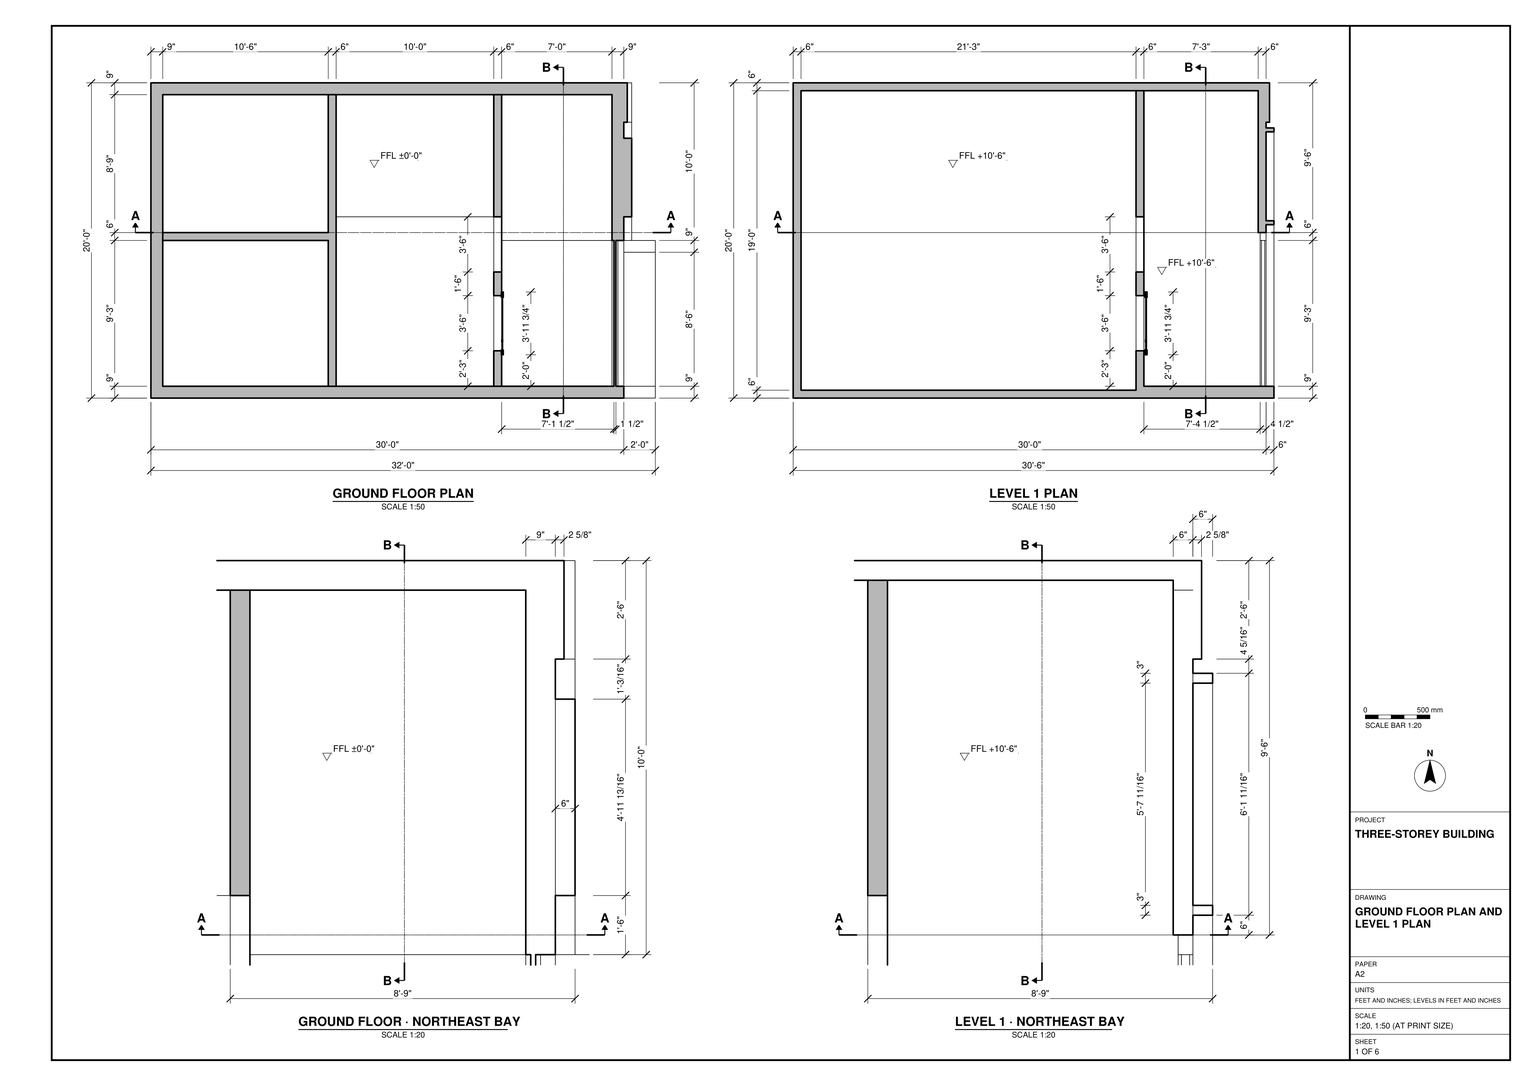
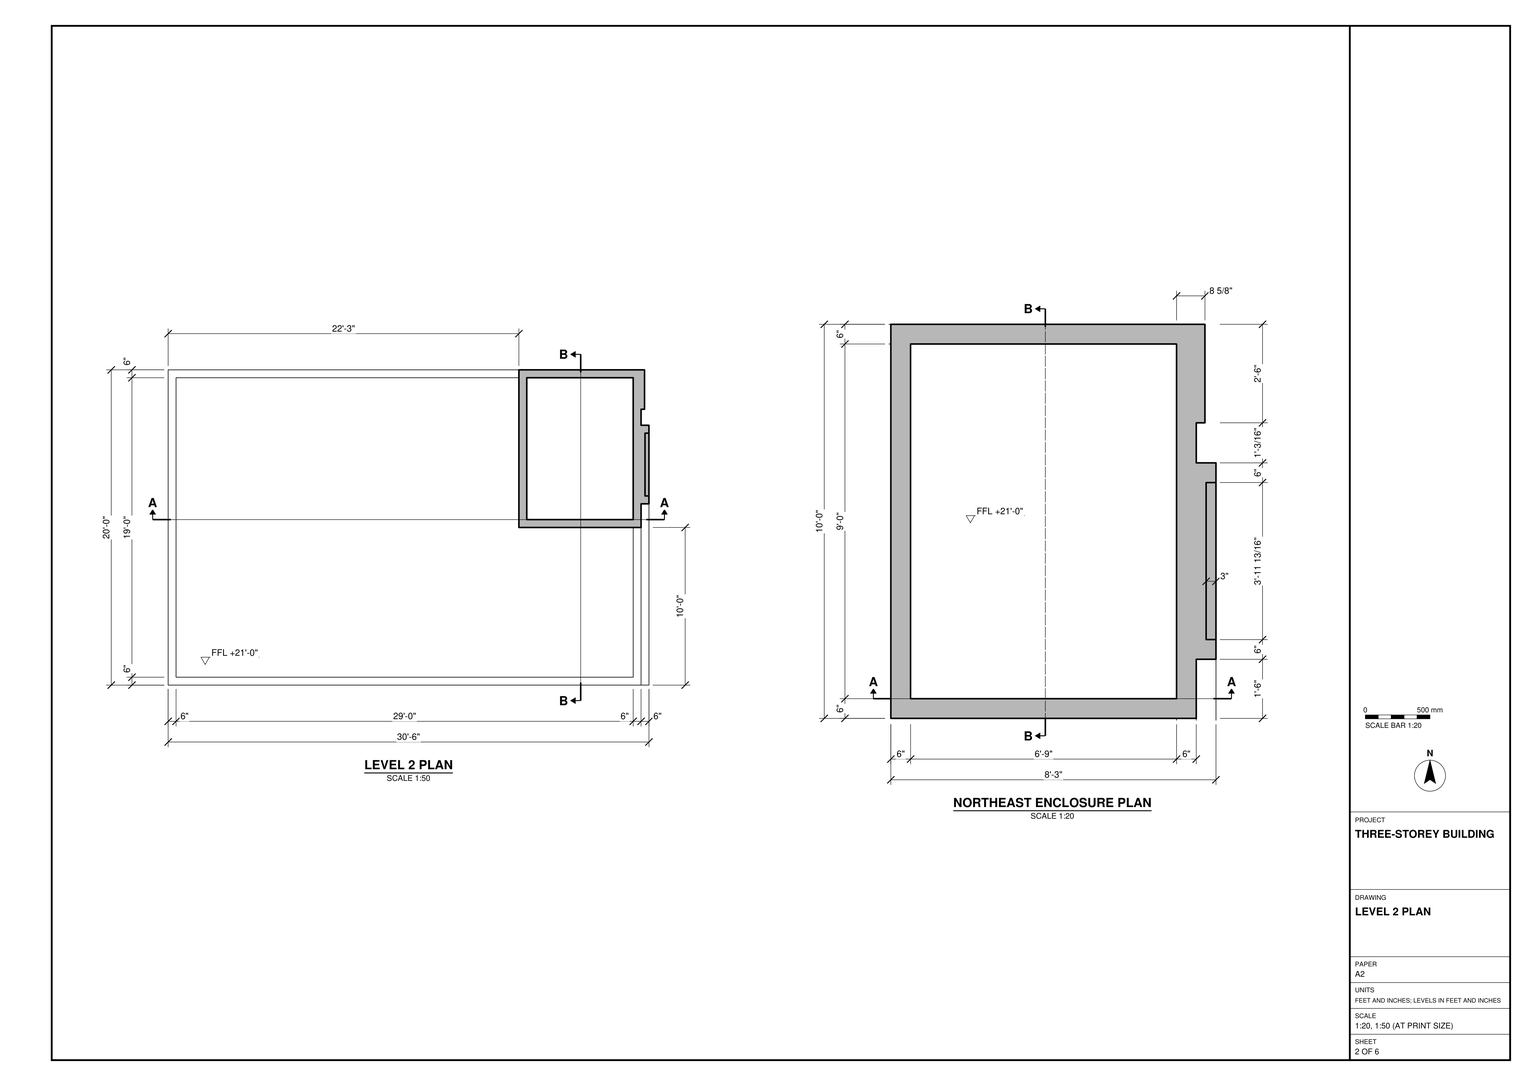
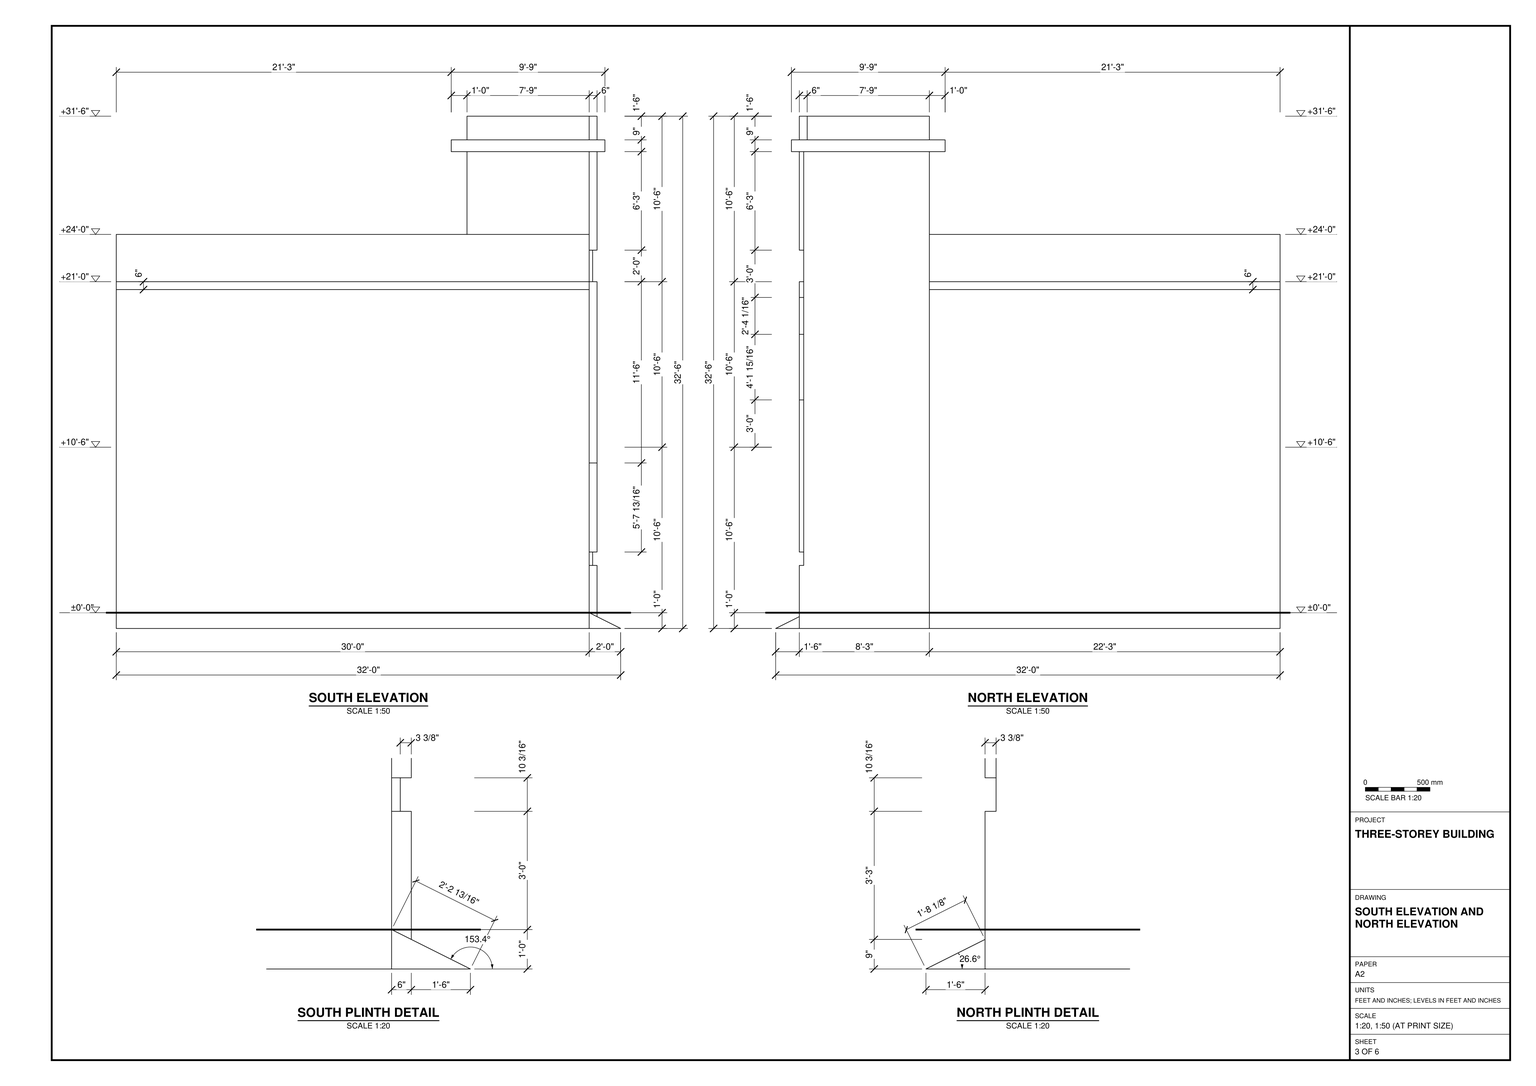
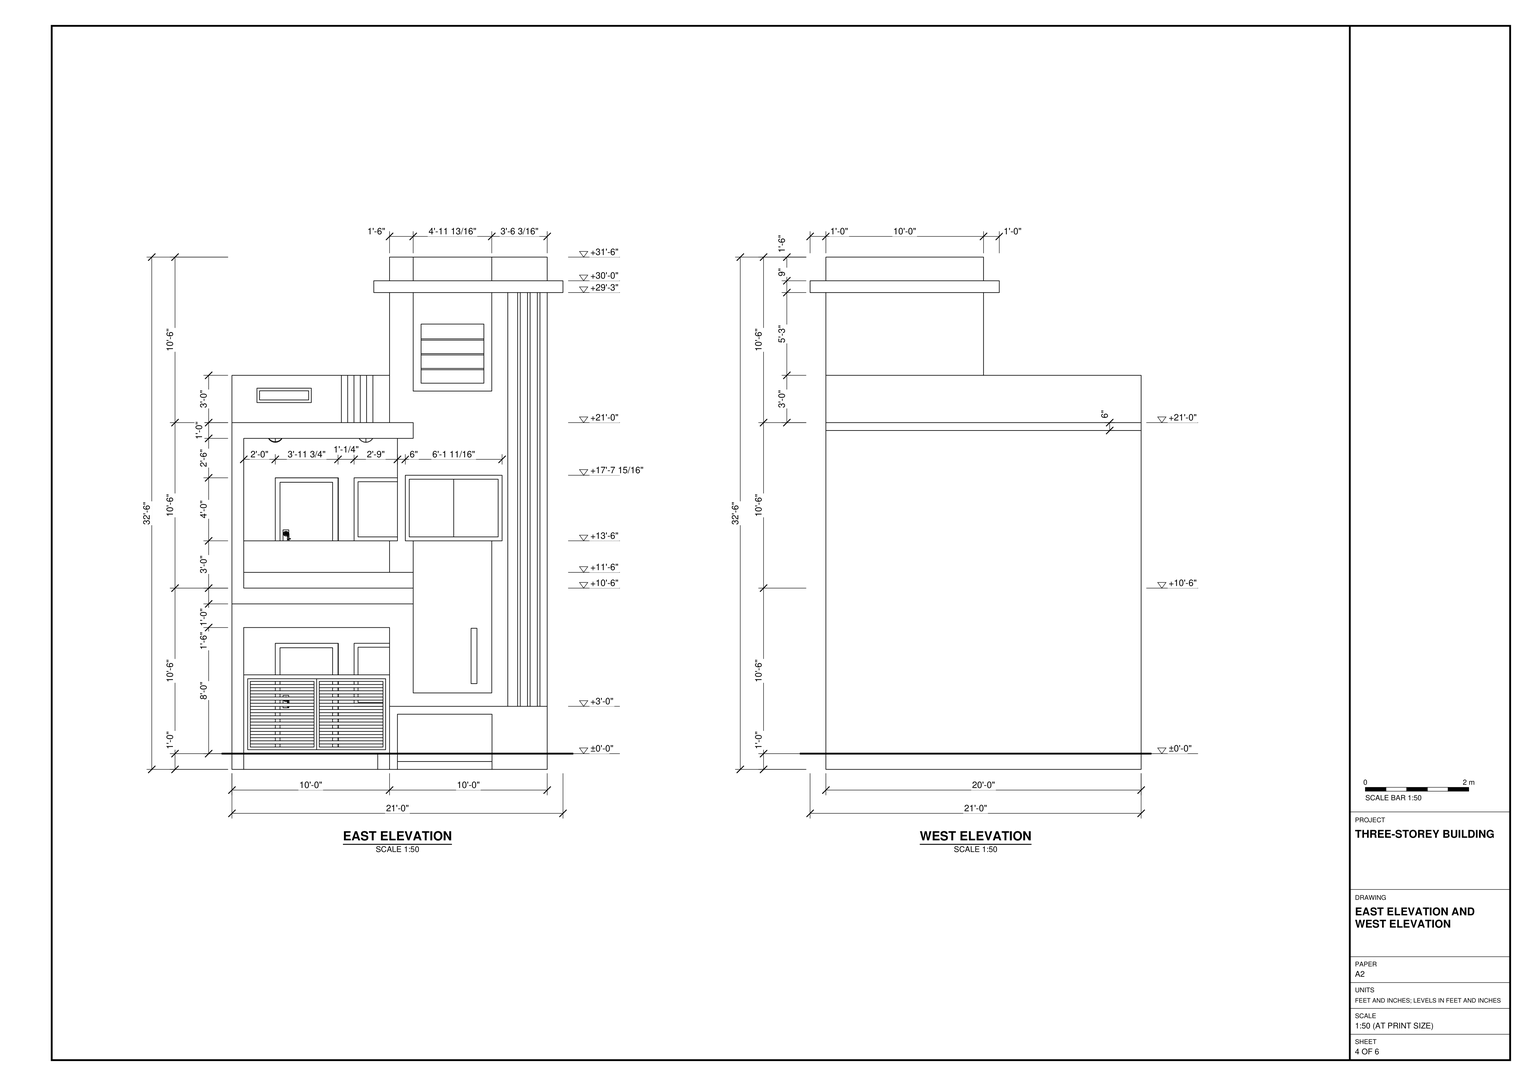
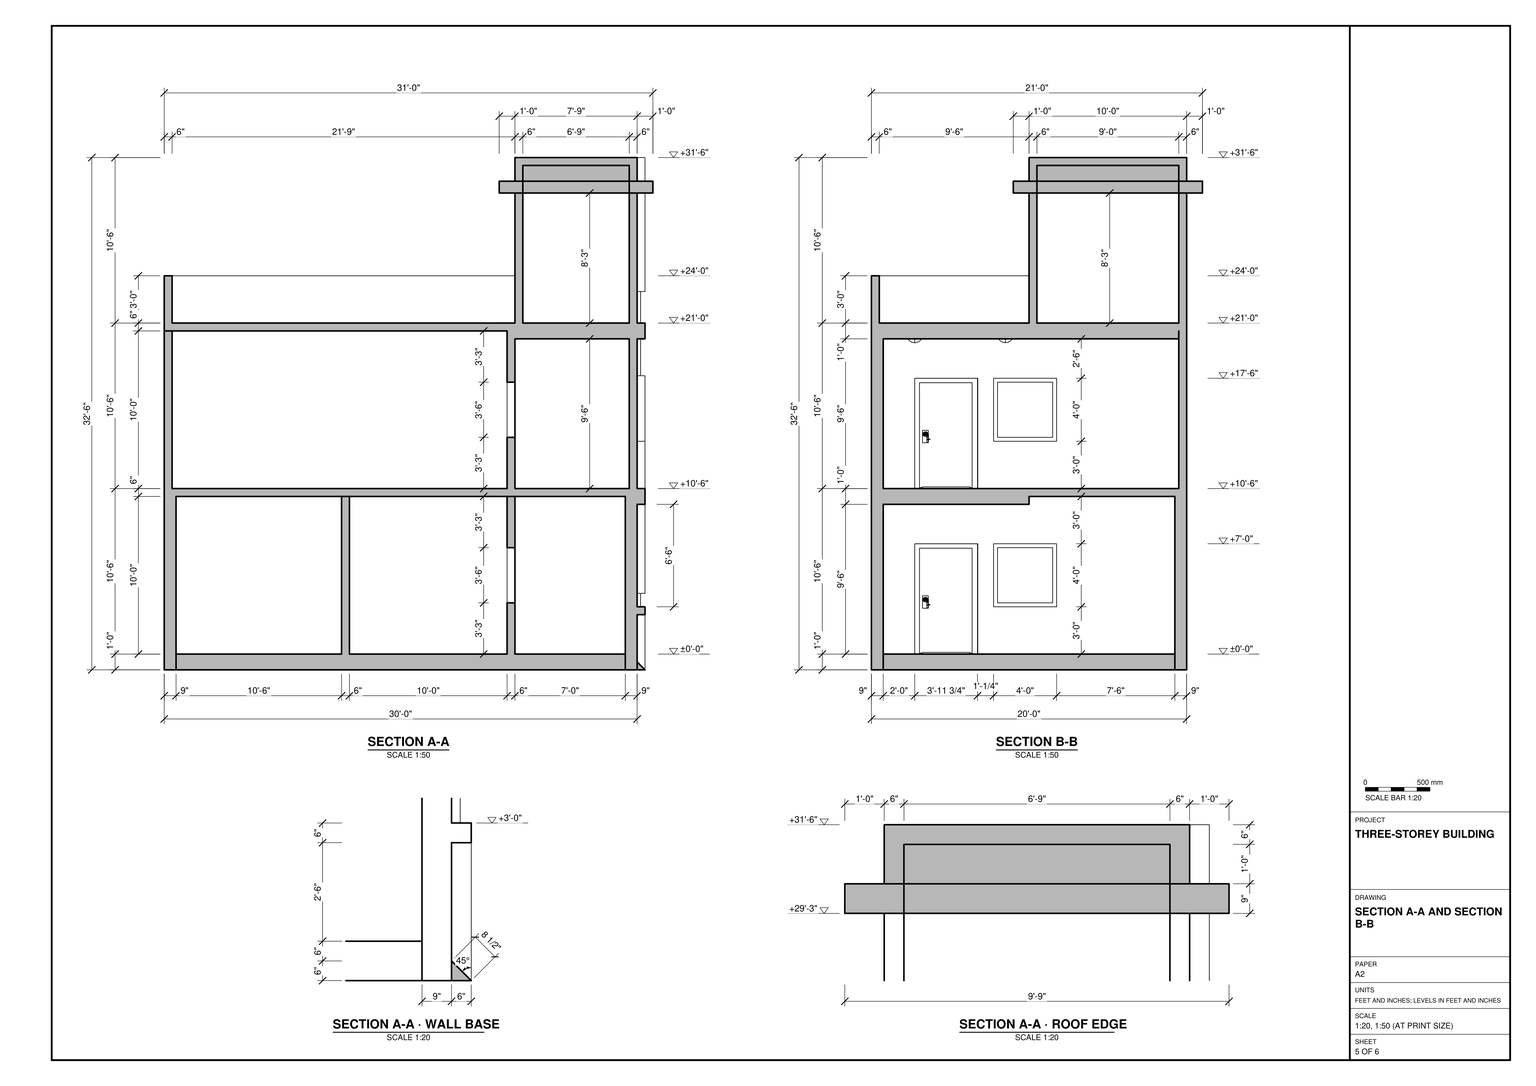
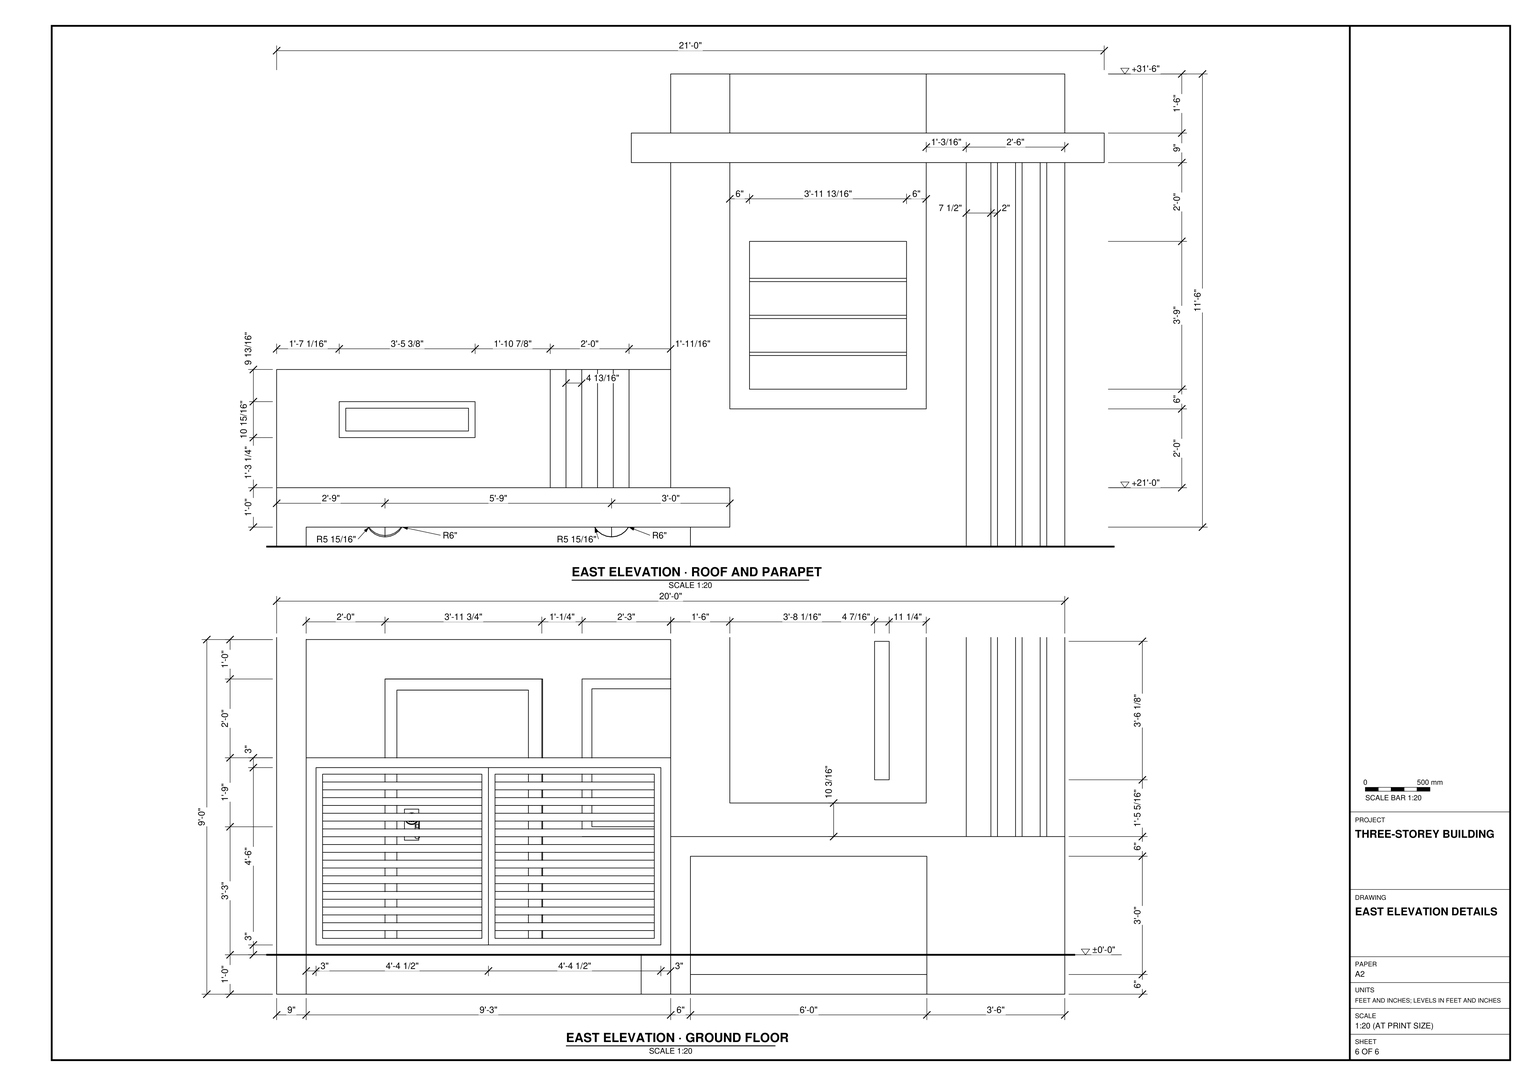
Build the three-storey building in SketchUp from task_files/diagram_01.pdf. Work in feet and inches. The overall extents, including the projecting plinth and roof edges, are 32'-0" along X, 21'-0" along Y and 32'-6" along Z. Set the finished floor levels at ±0'-0", +10'-6" and +21'-0". Measure the overall height from the underside of the plinth rather than from the ground floor.

Lay out the ground floor in three bays, with a cross wall dividing the west bay. On Level 1, leave the west space open and retain the narrow east bay. Follow the plans for wall thicknesses and opening positions, using the enlarged northeast bay drawings to resolve the wall profiles. Model the floor slabs and the sloping plinth projection. At Level 2, form the terrace with its perimeter parapet and place the roofed enclosure in the northeast corner. Match its stepped east face and projecting roof band to the plan and elevations.

Keep walls, slabs and roof elements in separate groups or components. Do the same for each furniture or joinery piece shown, and use components for repeated parts. Decor and loose items, where shown, may be any suitable library components. Save one SketchUp model as output_files/three_storey_building_with_northeast_rooftop_enclosure.skp.

# SketchUp Ruby script. Lengths in inches.
U = 1.inch
M = Sketchup.active_model
def pt(a) = Geom::Point3d.new(a.map { |v| v * U })
def face(e, loops, mat)
  f = e.add_face(loops[0].map { |a| pt(a) })
  loops[1..].each { |l| e.add_face(l.map { |a| pt(a) }).erase! }
  f.material = f.back_material = mat if mat
  f
end
# faces: each face lists its corners as indices into pts; further lists are holes
def faces(e, pts, list, mat = nil) = list.each { |f| face(e, (f[0].is_a?(Array) ? f : [f]).map { |l| l.map { |i| pts[i] } }, mat) }
# xy, xz, yz: faces in a plane at the given z, y or x. An outline is a flat list of corners, or four numbers for a rectangle; further outlines are holes
def ring(l) = l.size == 4 ? [[l[0], l[1]], [l[2], l[1]], [l[2], l[3]], [l[0], l[3]]] : l.each_slice(2).to_a
def flat(e, list, mat, &to3) = list.each { |f| face(e, (f[0].is_a?(Array) ? f : [f]).map { |l| ring(l).map { |u, v| to3.(u, v) } }, mat) }
def xy(e, z, list, mat = nil) = flat(e, list, mat) { |x, y| [x, y, z] }
def xz(e, y, list, mat = nil) = flat(e, list, mat) { |x, z| [x, y, z] }
def yz(e, x, list, mat = nil) = flat(e, list, mat) { |y, z| [x, y, z] }
def lines(e, pts, list) = list.each { |a, b| e.add_line(pt(pts[a]), pt(pts[b])) }
# prism: a flat outline (further loops are holes) pulled along v
def prism(e, loops, v, mat = nil)
  f = face(e, loops, mat); d = Geom::Vector3d.new(v.map { |x| x * U })
  f.pushpull(f.normal.samedirection?(d) ? d.length : -d.length)
end
def box(e, o, s, mat = nil) = prism(e, [[o, [o[0] + s[0], o[1], o[2]], [o[0] + s[0], o[1] + s[1], o[2]], [o[0], o[1] + s[1], o[2]]]], [0, 0, s[2]], mat)
def at(x, y, z, deg = 0) = Geom::Transformation.translation(pt([x, y, z])) * Geom::Transformation.rotation(ORIGIN, Z_AXIS, deg.degrees)
def axes(o, x, y, z) = Geom::Transformation.new([*x, 0, *y, 0, *z, 0, *pt(o).to_a, 1])
def part(name) = M.definitions.add(name)
# library, detail: a bought-in or finely detailed component or shape, given as its bounding box
def library(name, o, s) = part(name).tap { |d| box(d.entities, o, s) }
def detail(e, o, s) = box(e.add_group.entities, o, s)
def put(e, d, t, mat = nil) = e.add_instance(d, t).tap { |i| i.material = mat if mat }
def group(e, t, mat = nil) = e.add_group.tap { |g| g.transformation = t; g.material = mat if mat }.entities
root = M.entities
M.materials.add("Carpet_04_1K").color = [72, 139, 201]
M.materials.add("Glass_Basic_01").color = [255, 222, 91]
M.materials["Glass_Basic_01"].alpha = 0.67
M.materials.add("Glass_Basic_1").color = [33, 186, 36]
M.materials["Glass_Basic_1"].alpha = 0.55
M.materials.add("Glass_Basic_2").color = [161, 173, 186]
M.materials["Glass_Basic_2"].alpha = 0.25
M.materials.add("L02_Bubblegum_Pop").color = [255, 153, 204]
M.materials.add("M00_Soft_Cloud").color = [255, 255, 255]
M.materials.add("M04_Stone_Frost").color = [142, 142, 142]
M.materials.add("M06_Steel_Smoke").color = [86, 86, 86]
M.materials.add("M08_Obsidian_Black").color = [30, 30, 30]
M.materials.add("Plywood_08_1K").color = [173, 110, 26]
M.materials.add("Roofing_02_1K").color = [209, 255, 159]
M.materials.add("ThomThom - Waistcoat1").color = [155, 155, 155]
M.materials.add("[Wood_Cherry_Original]1").color = [76, 43, 21]
c1 = library("porta+4",[0.2,-5.42,1.33],[46.55,4.72,83.21])
c2 = library("Sphere Light",[-6,-6,-6],[12,12,12])
c3 = library("Sphere Light\#1",[-6,-6,-6],[12,12,12])
c4 = library("Sphere Light\#2",[-6,-6,-6],[12,12,12])
c5 = library("Sphere Light\#3",[-5.95,-5.95,-5.95],[11.9,11.9,11.9])
g1 = group(root,at(0,0,0))
box(g1,[273,126,264],[81,108,120])
xy(g1,0,[[[0,0,0,240,366,240,366,198,360,198,360,126,366,126,366,120,360,120,360,0],[9,9,351,231]],[360,0,384,9],[9,9,351,231],[360,9,384,111],[360,111,384,120]])
xy(g1,0,[[360,126,366,198]],"Roofing_02_1K")
xy(g1,12,[[9,9,135,120],[141,9,261,138],[267,9,351,120],[351,9,352.5,120],[354,9,355.5,120],
  [355.5,9,360,120],[267,120,351,231],[9,126,135,231],[141,138,261,231]])
xy(g1,15,[[261,36,267,78]])
xy(g1,17,[[352.5,14,354,62.5],[352.5,66.5,354,115]])
xy(g1,19.38,[[352.5,14,354,62.5],[352.5,66.5,354,115]])
xy(g1,21.76,[[352.5,14,354,62.5],[352.5,66.5,354,115]])
xy(g1,24.14,[[352.5,14,354,62.5],[352.5,66.5,354,115]])
xy(g1,26.52,[[352.5,14,354,62.5],[352.5,66.5,354,115]])
xy(g1,28.9,[[352.5,14,354,62.5],[352.5,66.5,354,115]])
xy(g1,31.29,[[352.5,14,354,62.5],[352.5,66.5,354,115]])
xy(g1,33.67,[[352.5,14,354,62.5],[352.5,66.5,354,115]])
xy(g1,36.05,[[352.5,14,354,62.5],[352.5,66.5,354,115]])
xy(g1,38.43,[[352.5,14,354,62.5],[352.5,66.5,354,115]])
xy(g1,40.81,[[352.5,14,354,62.5],[352.5,66.5,354,115]])
xy(g1,42,[[360,126,366,198]])
xy(g1,43.19,[[352.5,14,354,62.5],[352.5,66.5,354,115]])
xy(g1,45.57,[[352.5,14,354,62.5],[352.5,66.5,354,115]])
xy(g1,47.95,[[352.5,14,354,62.5],[352.5,66.5,354,115]])
xy(g1,48,[[360,120,366,210],[362.64,210,366,240]])
xy(g1,50.33,[[352.5,14,354,62.5],[352.5,66.5,354,115]])
xy(g1,51,[[261,96,267,138]])
xy(g1,52.71,[[352.5,14,354,62.5],[352.5,66.5,354,115]])
xy(g1,55.1,[[352.5,14,354,62.5],[352.5,66.5,354,115]])
xy(g1,57.48,[[352.5,14,354,62.5],[352.5,66.5,354,115]])
xy(g1,58.22,[[360,138,366,197.81]],"L02_Bubblegum_Pop")
xy(g1,59.86,[[352.5,14,354,62.5],[352.5,66.5,354,115]])
xy(g1,62.24,[[352.5,14,354,62.5],[352.5,66.5,354,115]])
xy(g1,64.62,[[352.5,14,354,62.5],[352.5,66.5,354,115]])
xy(g1,65.29,[[363,182.07,366,186.53]])
xy(g1,67,[[352.5,14,354,62.5],[352.5,66.5,354,115]])
xy(g1,72,[[352.5,9,354,120]])
xy(g1,93,[[261,36,267,78],[261,96,267,138]])
xy(g1,107.45,[[363,182.07,366,186.53]])
xy(g1,108,[[351,9,360,120]])
xy(g1,126,[[360,0,366,138],[267,9,351,120]])
xy(g1,132,[[9,9,135,120],[135,9,141,120],[141,9,261,138],[261,9,267,120],[9,120,141,126],
  [261,120,267,126],[267,120,351,126],[9,126,135,231],[135,126,141,231],[261,126,267,231],
  [267,126,351,231],[141,138,261,231]])
xy(g1,138,[[6,6,261,234],[267,9,355.5,9,355.5,126,354,126,354,234,267,234],[360,9,366,138]])
xy(g1,141,[[261,36,267,78]])
xy(g1,150,[[355.5,9,356.5,120],[359,9,360,120]])
xy(g1,174,[[356.5,9,359,120],[355.5,120,360,126],[360,132,366,138],[360,197.81,366,205.67]])
xy(g1,177,[[261,96,267,138],[360,135,366,202.67]])
xy(g1,219,[[261,36,267,78],[261,96,267,138]])
xy(g1,220.91,[[360,135,366,202.67]])
xy(g1,223.91,[[360,132,366,205.67]])
xy(g1,252,[[[267,9,267,126,360,126,360,138,366,138,366,9],[342,27,343.55,27.2,345,27.8,346.24,28.76,347.2,30,347.8,31.45,348,33,347.8,34.55,347.2,36,346.24,37.24,345,38.2,343.55,38.8,342,39,340.45,38.8,339,38.2,337.76,37.24,336.8,36,336.2,34.55,336,33,336.2,31.45,336.8,30,337.76,28.76,339,27.8,340.45,27.2],[291,96,292.55,96.2,294,96.8,295.24,97.76,296.2,99,296.8,100.45,297,102,296.8,103.55,296.2,105,295.24,106.24,294,107.2,292.55,107.8,291,108,289.45,107.8,288,107.2,286.76,106.24,285.8,105,285.2,103.55,285,102,285.2,100.45,285.8,99,286.76,97.76,288,96.8,289.45,96.2],[290.55,27.02,292.11,27.1,293.6,27.59,294.91,28.45,295.96,29.62,296.66,31.02,296.98,32.55,296.96,33,296.9,34.11,296.41,35.6,295.55,36.91,294.38,37.96,292.98,38.66,291.45,38.98,291,38.96,289.89,38.9,288.4,38.41,287.09,37.55,286.04,36.38,285.34,34.98,285.02,33.45,285.1,31.89,285.59,30.4,286.45,29.09,287.62,28.04,289.02,27.34],[342.1875,96,343.74,96.26,345.16,96.9,346.375,97.89,347.29,99.17,347.84,100.63,348,102.1875,347.74,103.74,347.1,105.16,346.11,106.375,344.83,107.29,343.37,107.84,341.8125,108,340.26,107.74,338.84,107.1,337.625,106.11,336.71,104.83,336.16,103.37,336.02,102,336,101.8125,336.26,100.26,336.9,98.84,337.89,97.625,339.17,96.71,340.63,96.16,342,96.02]],[267,126,354,234]])
xy(g1,255,[[290.55,27.02,289.02,27.34,287.62,28.04,286.45,29.09,285.59,30.4,285.1,31.89,285.02,33.45,285.34,34.98,286.04,36.38,287.09,37.55,288.4,38.41,289.89,38.9,291,38.96,291,33,296.96,33,296.98,32.55,296.66,31.02,295.96,29.62,294.91,28.45,293.6,27.59,292.11,27.1],[291,33,291,38.96,291.45,38.98,292.98,38.66,294.38,37.96,295.55,36.91,296.41,35.6,296.9,34.11,296.96,33],[291,96,289.45,96.2,288,96.8,286.76,97.76,285.8,99,285.2,100.45,285,102,285.2,103.55,285.8,105,286.76,106.24,288,107.2,289.45,107.8,291,108,292.55,107.8,294,107.2,295.24,106.24,296.2,105,296.8,103.55,297,102,291,102],[291,96,291,102,297,102,296.8,100.45,296.2,99,295.24,97.76,294,96.8,292.55,96.2],[342.1875,96,342,96.02,342,102,336.02,102,336.16,103.37,336.71,104.83,337.625,106.11,338.84,107.1,340.26,107.74,341.8125,108,343.37,107.84,344.83,107.29,346.11,106.375,347.1,105.16,347.74,103.74,348,102.1875,347.84,100.63,347.29,99.17,346.375,97.89,345.16,96.9,343.74,96.26],
  [342,96.02,340.63,96.16,339.17,96.71,337.89,97.625,336.9,98.84,336.26,100.26,336,101.8125,336.02,102,342,102]])
xy(g1,255.42,[[342,27,340.45,27.2,339,27.8,337.76,28.76,336.8,30,336.2,31.45,336,33,342,33,342,39,343.55,38.8,345,38.2,346.24,37.24,347.2,36,347.8,34.55,348,33,347.8,31.45,347.2,30,346.24,28.76,345,27.8,343.55,27.2],[336,33,336.2,34.55,336.8,36,337.76,37.24,339,38.2,340.45,38.8,342,39,342,33]])
xy(g1,258,[[0,0,267,6],[0,6,6,240],[6,6,261,234]])
xy(g1,264,[[360,0,366,138],[6,6,354,6,354,120,267,120,267,234,6,234]])
xy(g1,281.26,[[354,21.05,360,58.43]])
xy(g1,288,[[360,138,366,197.81]])
xy(g1,288.21,[[354,21.05,360,58.43]])
xy(g1,294,[[363,144,366,191.81]],"L02_Bubblegum_Pop")
xy(g1,300,[[0,0,360,0,360,120,354,120,354,6,6,6,6,234,267,234,267,240,0,240]])
xy(g1,304.25,[[363,144,366,191.81]],"L02_Bubblegum_Pop")
xy(g1,305.25,[[363,144,366,191.81]],"L02_Bubblegum_Pop")
xy(g1,315.51,[[363,144,366,191.81]],"L02_Bubblegum_Pop")
xy(g1,316.51,[[363,144,366,191.81]],"L02_Bubblegum_Pop")
xy(g1,326.76,[[363,144,366,191.81]],"L02_Bubblegum_Pop")
xy(g1,327.76,[[363,144,366,191.81]],"L02_Bubblegum_Pop")
xy(g1,339.02,[[363,144,366,191.81]],"L02_Bubblegum_Pop")
xy(g1,363,[[255,108,255,120,360,120,360,138,366,138,366,197.81,360,197.81,360,210,362.64,210,362.64,252,372,252,372,108],[255,120,267,252],[267,120,360,120,360,138,366,138,366,197.81,360,197.81,360,210,362.64,210,362.64,240,267,240],[267,240,362.64,252]])
xy(g1,372,[[[255,108,372,252],[267,120,267,240,360,240,360,197.81,366,197.81,366,138,360,138,360,120]],[267,120,267,240,360,240,360,197.81,366,197.81,366,138,360,138,360,120]])
xy(g1,390,[[267,120,360,240]],"Carpet_04_1K")
xy(g1,390,[[360,138,366,197.81]],"L02_Bubblegum_Pop")
xz(g1,0,[[0,0,360,258],[360,0,384,0,360,12],[360,126,366,264],[0,258,360,264],[0,264,360,300]])
xz(g1,6,[[6,138,261,258],[6,264,354,300]])
xz(g1,9,[[9,0,261,12],[261,0,267,12],[267,0,351,12],[360,0,360,12,384,0],[9,12,135,132],
  [135,12,141,132],[141,12,261,132],[261,12,267,132],[267,12,267,126,351,126,351,108,360,108,360,12,354,12,354,72,352.5,72,352.5,12],[267,138,267,252,366,252,366,138,360,138,360,150,359,150,359,174,356.5,174,356.5,150,355.5,150,355.5,138]])
xz(g1,14,[[352.5,17,354,19.38],[352.5,21.76,354,24.14],[352.5,26.52,354,28.9],[352.5,31.29,354,33.67],[352.5,36.05,354,38.43],
  [352.5,40.81,354,43.19],[352.5,45.57,354,47.95],[352.5,50.33,354,52.71],[352.5,55.1,354,57.48],[352.5,59.86,354,62.24],
  [352.5,64.62,354,67]])
xz(g1,21.05,[[354,281.26,360,288.21]])
xz(g1,36,[[261,15,267,93],[261,141,267,219]])
xz(g1,58.43,[[354,281.26,360,288.21]])
xz(g1,62.5,[[352.5,17,354,19.38],[352.5,21.76,354,24.14],[352.5,26.52,354,28.9],[352.5,31.29,354,33.67],[352.5,36.05,354,38.43],
  [352.5,40.81,354,43.19],[352.5,45.57,354,47.95],[352.5,50.33,354,52.71],[352.5,55.1,354,57.48],[352.5,59.86,354,62.24],
  [352.5,64.62,354,67]])
xz(g1,66.5,[[352.5,17,354,19.38],[352.5,21.76,354,24.14],[352.5,26.52,354,28.9],[352.5,31.29,354,33.67],[352.5,36.05,354,38.43],
  [352.5,40.81,354,43.19],[352.5,45.57,354,47.95],[352.5,50.33,354,52.71],[352.5,55.1,354,57.48],[352.5,59.86,354,62.24],
  [352.5,64.62,354,67]])
xz(g1,78,[[261,15,267,93],[261,141,267,219]])
xz(g1,96,[[261,51,267,93],[261,177,267,219]])
xz(g1,108,[[255,363,372,372]])
xz(g1,111,[[360,0,384,0,360,12]])
xz(g1,115,[[352.5,17,354,19.38],[352.5,21.76,354,24.14],[352.5,26.52,354,28.9],[352.5,31.29,354,33.67],[352.5,36.05,354,38.43],
  [352.5,40.81,354,43.19],[352.5,45.57,354,47.95],[352.5,50.33,354,52.71],[352.5,55.1,354,57.48],[352.5,59.86,354,62.24],
  [352.5,64.62,354,67]])
xz(g1,120,[[360,0,366,0,366,9,360,12],[366,0,384,0,366,9],[366,9,366,12,360,12],[9,12,135,132],[351,12,352.5,12,352.5,72,354,72,354,12,366,12,366,48,360,48,360,108,351,108],
  [267,126,351,132],[355.5,150,356.5,174],[359,150,360,174]])
xz(g1,120,[[267,264,354,264,354,300,360,300,360,363,267,363],[267,372,360,390]],"Carpet_04_1K")
xz(g1,126,[[360,0,360,6,366,0],[366,0,360,6,360,42,366,42],[9,12,135,132],[354,138,355.5,138,355.5,174,360,174,360,252,354,252]])
xz(g1,132,[[360,174,366,223.91]])
xz(g1,135,[[360,177,366,220.91]])
xz(g1,138,[[261,51,267,93],[261,177,267,219],[360,252,366,264]])
xz(g1,138,[[360,58.22,366,126],[360,138,366,174],[360,288,366,363],[360,372,366,390]],"L02_Bubblegum_Pop")
xz(g1,144,[[363,294,366,304.25],[363,305.25,366,315.51],[363,316.51,366,326.76],[363,327.76,366,339.02]],"L02_Bubblegum_Pop")
xz(g1,182.07,[[363,65.29,366,107.45]])
xz(g1,186.53,[[363,65.29,366,107.45]])
xz(g1,191.81,[[363,294,366,304.25],[363,305.25,366,315.51],[363,316.51,366,326.76],[363,327.76,366,339.02]],"L02_Bubblegum_Pop")
xz(g1,197.81,[[360,58.22,366,174],[360,288,366,363],[360,372,366,390]],"L02_Bubblegum_Pop")
xz(g1,198,[[360,0,366,0,360,6],[366,0,366,42,360,42,360,6]])
xz(g1,202.67,[[360,177,366,220.91]])
xz(g1,205.67,[[360,174,366,223.91]])
xz(g1,210,[[360,48,362.64,363]])
xz(g1,231,[[9,0,261,0,261,12,141,12,141,132,135,132,135,12,9,12],[261,0,267,132],[267,0,351,12],[9,12,135,132],[141,12,261,132],
  [267,12,351,132]])
xz(g1,234,[[6,138,261,258],[261,138,261,258,354,258,354,252,267,252,267,138],[267,138,354,252],[6,264,267,300]])
xz(g1,240,[[0,0,267,258],[0,258,267,264],[0,264,267,300]])
xz(g1,240,[[267,0,267,363,362.64,363,362.64,48,366,48,366,0],[267,372,360,390]],"Carpet_04_1K")
xz(g1,252,[[255,363,372,372]])
yz(g1,0,[[0,0,240,258],[0,258,240,264],[0,264,240,300]])
yz(g1,6,[[6,138,234,258],[6,264,234,300]])
yz(g1,9,[[9,0,120,12],[120,0,126,132],[126,0,231,12],[9,12,120,132],[126,12,231,132]])
yz(g1,135,[[9,12,120,132],[126,12,231,132]])
yz(g1,141,[[9,12,138,132],[138,12,231,132]])
yz(g1,255,[[108,363,252,372]])
yz(g1,261,[[[9,12,9,132,138,132,138,93,96,93,96,51,138,51,138,12],[36,15,78,93]],[138,12,231,132],[[6,138,234,258],[36,141,78,219],[96,177,138,219]]])
yz(g1,267,[[[9,12,33,12,33,96,81,96,81,12,231,12,231,132,120,132,120,126,9,126],[93,48,141,96]],[[33,12,81,96],[36,15,78,93]],[9,126,120,132],[[9,138,33,138,33,222,81,222,81,138,234,138,234,252,9,252],[93,174,141,222]],[[33,138,81,222],[36,141,78,219]]])
yz(g1,267,[[120,264,120,363,240,363,240,300,234,300,234,264],[120,372,240,390]],"Carpet_04_1K")
yz(g1,267,[[96,51,138,93],[96,177,138,219]],"Glass_Basic_01")
yz(g1,267,[[[93,48,141,96],[96,51,138,93]],[[93,174,141,222],[96,177,138,219]]],"[Wood_Cherry_Original]1")
yz(g1,351,[[9,0,231,12],[120,12,231,132],[9,108,120,126]])
yz(g1,352.5,[[[9,12,120,72],[14,17,62.5,19.38],[66.5,17,115,19.38],[14,50.33,62.5,52.71],[66.5,50.33,115,52.71],[14,64.62,62.5,67],[14,59.86,62.5,62.24],[14,55.1,62.5,57.48],[14,45.57,62.5,47.95],[14,40.81,62.5,43.19],[14,36.05,62.5,38.43],[14,31.29,62.5,33.67],[14,26.52,62.5,28.9],[14,21.76,62.5,24.14],[66.5,64.62,115,67],[66.5,59.86,115,62.24],[66.5,55.1,115,57.48],[66.5,45.57,115,47.95],[66.5,40.81,115,43.19],[66.5,36.05,115,38.43],[66.5,31.29,115,33.67],[66.5,26.52,115,28.9],[66.5,21.76,115,24.14]]])
yz(g1,354,[[126,138,234,252],[[6,264,120,300],[21.05,281.26,58.43,288.21]]])
yz(g1,354,[[14,19.38,62.5,21.76],[66.5,19.38,115,21.76],[14,24.14,62.5,26.52],[66.5,24.14,115,26.52],[14,28.9,62.5,31.29],
  [66.5,28.9,115,31.29],[14,33.67,62.5,36.05],[66.5,33.67,115,36.05],[14,38.43,62.5,40.81],[66.5,38.43,115,40.81],
  [14,43.19,62.5,45.57],[66.5,43.19,115,45.57],[14,47.95,62.5,50.33],[66.5,47.95,115,50.33],[14,52.71,62.5,55.1],
  [66.5,52.71,115,55.1],[14,57.48,62.5,59.86],[66.5,57.48,115,59.86],[14,62.24,62.5,64.62],[66.5,62.24,115,64.62]],"M00_Soft_Cloud")
yz(g1,354,[[[9,12,120,72],[12,15,117,69]],[[12,15,64.5,69],[14,17,62.5,67]],[[64.5,15,117,69],[66.5,17,115,67]]],"M08_Obsidian_Black")
yz(g1,355.5,[[9,138,120,150],[120,138,126,174]])
yz(g1,356.5,[[9,150,120,174]],"Glass_Basic_2")
yz(g1,359,[[9,150,120,174]],"Glass_Basic_2")
yz(g1,360,[[0,0,9,12],[9,0,111,12],[111,0,120,12],[[0,264,83.32,300],[19.05,279.26,60.43,290.21]],[88.12,264,92.92,300],
  [97.72,264,102.52,300],[107.32,264,120,300],[[19.05,279.26,60.43,290.21],[21.05,281.26,58.43,288.21]]])
yz(g1,360,[[0,12,9,12,9,108,120,108,120,48,210,48,210,363,197.81,363,197.81,288,138,288,138,363,120,363,120,264,138,264,138,252,126,252,126,174,120,174,120,150,138,150,138,174,132,174,132,223.91,205.67,223.91,205.67,174,197.81,174,197.81,58.22,138,58.22,138,126,0,126],[120,372,138,390],[197.81,372,240,390]],"Carpet_04_1K")
yz(g1,360,[[135,177,168.83,220.91]],"Glass_Basic_01")
yz(g1,360,[[83.32,264,88.12,300],[92.92,264,97.72,300],[102.52,264,107.32,300]],"M04_Stone_Frost")
yz(g1,360,[[126,0,198,6],[126,6,198,42],[9,138,138,150],[168.83,177,202.67,220.91]],"Plywood_08_1K")
yz(g1,362.64,[[217.5,48,219.5,363],[225,48,227,363],[232.5,48,234.5,363]],"M00_Soft_Cloud")
yz(g1,362.64,[[210,48,217.5,363],[219.5,48,225,363],[227,48,232.5,363],[234.5,48,240,363]],"M06_Steel_Smoke")
yz(g1,363,[[182.07,65.29,186.53,107.45]])
yz(g1,363,[[144,294,191.81,304.25],[144,305.25,191.81,315.51],[144,316.51,191.81,326.76],[144,327.76,191.81,339.02]],"L02_Bubblegum_Pop")
yz(g1,366,[[120,0,126,0,126,42,198,42,198,0,240,0,240,48,120,48],[0,126,138,126,138,138,9,138,9,252,138,252,138,264,0,264],[[132,174,205.67,223.91],[135,177,202.67,220.91]]])
yz(g1,366,[[144,294,191.81,304.25],[144,305.25,191.81,315.51],[144,316.51,191.81,326.76],[144,327.76,191.81,339.02]],"Glass_Basic_1")
yz(g1,366,[[[138,58.22,197.81,174],[182.07,65.29,186.53,107.45]],[[138,288,197.81,363],[144,294,191.81,339.02]],[144,304.25,191.81,305.25],[144,315.51,191.81,316.51],[144,326.76,191.81,327.76],
  [138,372,197.81,390]],"L02_Bubblegum_Pop")
yz(g1,372,[[108,363,252,372]])
p = [[360,0,12],[384,0,0],[384,9,0],[360,9,12],[384,111,0],[360,111,12],
  [384,120,0],[366,120,9],[360,120,12],[366,198,0],[360,198,6],[360,126,6],
  [366,126,0],[290.55,27.02,252],[289.02,27.34,252],[289.02,27.34,255],[290.55,27.02,255],[292.11,27.1,252],
  [292.11,27.1,255],[342,27,252],[340.45,27.2,252],[340.45,27.2,255.42],[342,27,255.42],[343.55,27.2,252],
  [343.55,27.2,255.42],[293.6,27.59,252],[293.6,27.59,255],[339,27.8,252],[339,27.8,255.42],[345,27.8,252],
  [345,27.8,255.42],[287.62,28.04,252],[287.62,28.04,255],[294.91,28.45,252],[294.91,28.45,255],[337.76,28.76,252],
  [337.76,28.76,255.42],[346.24,28.76,252],[346.24,28.76,255.42],[286.45,29.09,252],[286.45,29.09,255],[295.96,29.62,252],
  [295.96,29.62,255],[336.8,30,252],[336.8,30,255.42],[347.2,30,252],[347.2,30,255.42],[285.59,30.4,252],
  [285.59,30.4,255],[296.66,31.02,252],[296.66,31.02,255],[336.2,31.45,252],[336.2,31.45,255.42],[347.8,31.45,252],
  [347.8,31.45,255.42],[285.1,31.89,252],[285.1,31.89,255],[296.98,32.55,252],[296.98,32.55,255],[336,33,252],
  [336,33,255.42],[348,33,252],[348,33,255.42],[285.02,33.45,252],[285.02,33.45,255],[296.96,33,252],
  [296.96,33,255],[296.9,34.11,252],[296.9,34.11,255],[336.2,34.55,252],[336.2,34.55,255.42],[347.8,34.55,252],
  [347.8,34.55,255.42],[285.34,34.98,252],[285.34,34.98,255],[296.41,35.6,252],[296.41,35.6,255],[336.8,36,252],
  [336.8,36,255.42],[347.2,36,252],[347.2,36,255.42],[286.04,36.38,252],[286.04,36.38,255],[295.55,36.91,252],
  [295.55,36.91,255],[337.76,37.24,252],[337.76,37.24,255.42],[346.24,37.24,252],[346.24,37.24,255.42],[287.09,37.55,252],
  [287.09,37.55,255],[294.38,37.96,252],[294.38,37.96,255],[339,38.2,252],[339,38.2,255.42],[345,38.2,252],
  [345,38.2,255.42],[288.4,38.41,252],[288.4,38.41,255],[292.98,38.66,252],[292.98,38.66,255],[340.45,38.8,252],
  [340.45,38.8,255.42],[343.55,38.8,252],[343.55,38.8,255.42],[289.89,38.9,252],[289.89,38.9,255],[291.45,38.98,252],
  [291.45,38.98,255],[342,39,252],[342,39,255.42],[291,38.96,252],[291,38.96,255],[291,96,252],
  [289.45,96.2,252],[289.45,96.2,255],[291,96,255],[292.55,96.2,252],[292.55,96.2,255],[342,96.02,252],
  [340.63,96.16,252],[340.63,96.16,255],[342,96.02,255],[342.1875,96,252],[342.1875,96,255],[343.74,96.26,252],
  [343.74,96.26,255],[288,96.8,252],[288,96.8,255],[294,96.8,252],[294,96.8,255],[339.17,96.71,252],
  [339.17,96.71,255],[345.16,96.9,252],[345.16,96.9,255],[337.89,97.625,252],[337.89,97.625,255],[286.76,97.76,252],
  [286.76,97.76,255],[295.24,97.76,252],[295.24,97.76,255],[346.375,97.89,252],[346.375,97.89,255],[336.9,98.84,252],
  [336.9,98.84,255],[285.8,99,252],[285.8,99,255],[296.2,99,252],[296.2,99,255],[347.29,99.17,252],
  [347.29,99.17,255],[336.26,100.26,252],[336.26,100.26,255],[285.2,100.45,252],[285.2,100.45,255],[296.8,100.45,252],
  [296.8,100.45,255],[347.84,100.63,252],[347.84,100.63,255],[336,101.8125,252],[336,101.8125,255],[285,102,252],
  [285,102,255],[297,102,252],[297,102,255],[348,102.1875,252],[348,102.1875,255],[336.02,102,252],
  [336.02,102,255],[285.2,103.55,252],[285.2,103.55,255],[296.8,103.55,252],[296.8,103.55,255],[336.16,103.37,252],
  [336.16,103.37,255],[347.74,103.74,252],[347.74,103.74,255],[336.71,104.83,252],[336.71,104.83,255],[285.8,105,252],
  [285.8,105,255],[296.2,105,252],[296.2,105,255],[347.1,105.16,252],[347.1,105.16,255],[337.625,106.11,252],
  [337.625,106.11,255],[286.76,106.24,252],[286.76,106.24,255],[295.24,106.24,252],[295.24,106.24,255],[346.11,106.375,252],
  [346.11,106.375,255],[338.84,107.1,252],[338.84,107.1,255],[288,107.2,252],[288,107.2,255],[294,107.2,252],
  [294,107.2,255],[344.83,107.29,252],[344.83,107.29,255],[340.26,107.74,252],[340.26,107.74,255],[289.45,107.8,252],
  [289.45,107.8,255],[292.55,107.8,252],[292.55,107.8,255],[343.37,107.84,252],[343.37,107.84,255],[341.8125,108,252],
  [341.8125,108,255],[291,108,252],[291,108,255],[354,126,258],[360,126,258],[9,231,132],
  [9,240,132],[354,234,258],[360,234,258],[267,9,132],[267,0,132],[351,231,132],
  [360,231,132],[351,126,132],[360,126,132],[267,120,252],[267,120,264],[273,126,384],
  [267,126,384],[354,126,384],[360,126,384],[273,234,384],[273,240,384],[354,234,384],
  [354,240,384],[267,0,252],[267,6,252],[267,6,258],[267,9,126],[267,0,126],
  [267,9,252]]
faces(g1,p,[[0,1,2,3],[3,2,4,5],[5,4,6,7,8]],"ThomThom - Waistcoat1")
faces(g1,p,[[9,10,11,12]],"Roofing_02_1K")
faces(g1,p,[[13,14,15,16],[17,13,16,18],[19,20,21,22],[23,19,22,24],[25,17,18,26],[20,27,28,21],[29,23,24,30],[14,31,32,15],
  [33,25,26,34],[27,35,36,28],[37,29,30,38],[31,39,40,32],[41,33,34,42],[35,43,44,36],[45,37,38,46],[39,47,48,40],
  [49,41,42,50],[43,51,52,44],[53,45,46,54],[47,55,56,48],[57,49,50,58],[51,59,60,52],[61,53,54,62],[55,63,64,56],
  [65,57,58,66],[67,65,66,68],[59,69,70,60],[71,61,62,72],[63,73,74,64],[75,67,68,76],[69,77,78,70],[79,71,72,80],
  [73,81,82,74],[83,75,76,84],[77,85,86,78],[87,79,80,88],[81,89,90,82],[91,83,84,92],[85,93,94,86],[95,87,88,96],
  [89,97,98,90],[99,91,92,100],[93,101,102,94],[103,95,96,104],[97,105,106,98],[107,99,100,108],[101,109,110,102],[109,103,104,110],
  [105,111,112,106],[111,107,108,112],[113,114,115,116],[117,113,116,118],[119,120,121,122],[123,119,122,124],[125,123,124,126],[114,127,128,115],
  [129,117,118,130],[120,131,132,121],[133,125,126,134],[131,135,136,132],[127,137,138,128],[139,129,130,140],[141,133,134,142],[135,143,144,136],
  [137,145,146,138],[147,139,140,148],[149,141,142,150],[143,151,152,144],[145,153,154,146],[155,147,148,156],[157,149,150,158],[151,159,160,152],
  [153,161,162,154],[163,155,156,164],[165,157,158,166],[159,167,168,160],[161,169,170,162],[171,163,164,172],[167,173,174,168],[175,165,166,176],
  [173,177,178,174],[169,179,180,170],[181,171,172,182],[183,175,176,184],[177,185,186,178],[179,187,188,180],[189,181,182,190],[191,183,184,192],
  [185,193,194,186],[187,195,196,188],[197,189,190,198],[199,191,192,200],[193,201,202,194],[195,203,204,196],[205,197,198,206],[207,199,200,208],
  [201,209,210,202],[203,211,212,204],[211,205,206,212],[209,207,208,210]])
lines(g1,p,[[213,214],[215,216],[217,218],[219,220],[221,222],[223,224],[225,226],[227,228],[229,230],[231,232],[233,234],[235,236],
  [237,236],[238,239],[236,240]])
put(g1,c1,axes([265.43,32.79,10.65],[0,1.026,0],[-0.57,0,0],[0,0,1.00974]))
put(g1,c1,axes([266.6,32.79,136.65],[0,1.026,0],[-0.57,0,0],[0,0,1.0096]))
put(g1,c2,at(342,33,255.42))
put(g1,c3,at(342,102,255))
put(g1,c4,at(291,33,255))
put(g1,c5,at(291,102,255))
